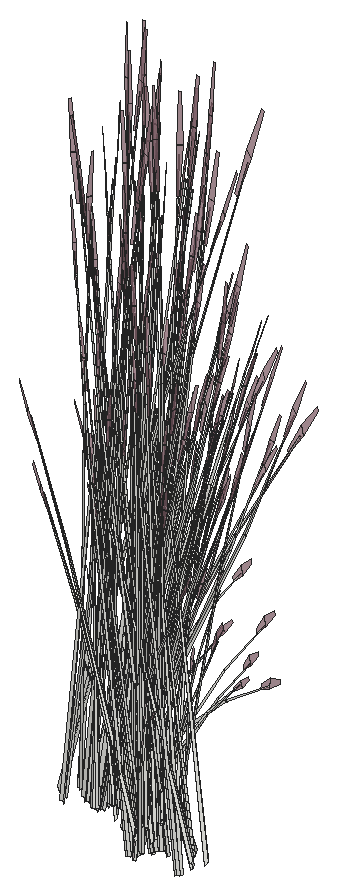
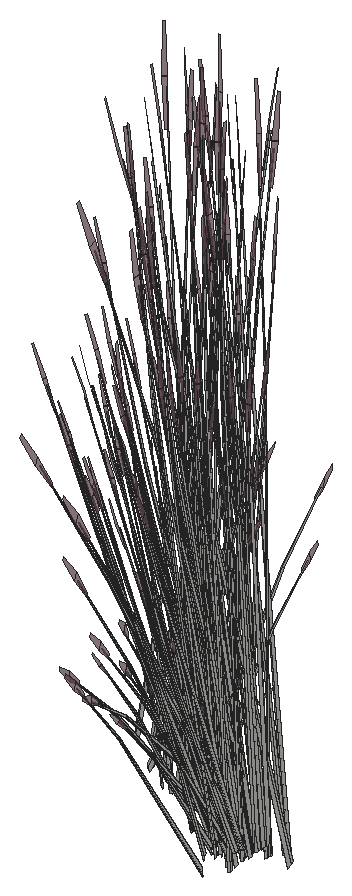
# SketchUp Ruby script. Lengths in inches.
U = 1.inch
M = Sketchup.active_model
def pt(a) = Geom::Point3d.new(a.map { |v| v * U })
def face(e, loops, mat)
  f = e.add_face(loops[0].map { |a| pt(a) })
  loops[1..].each { |l| e.add_face(l.map { |a| pt(a) }).erase! }
  f.material = f.back_material = mat if mat
  f
end
# faces: each face lists its corners as indices into pts; further lists are holes
def faces(e, pts, list, mat = nil) = list.each { |f| face(e, (f[0].is_a?(Array) ? f : [f]).map { |l| l.map { |i| pts[i] } }, mat) }
# xy, xz, yz: faces in a plane at the given z, y or x. An outline is a flat list of corners, or four numbers for a rectangle; further outlines are holes
def ring(l) = l.size == 4 ? [[l[0], l[1]], [l[2], l[1]], [l[2], l[3]], [l[0], l[3]]] : l.each_slice(2).to_a
def flat(e, list, mat, &to3) = list.each { |f| face(e, (f[0].is_a?(Array) ? f : [f]).map { |l| ring(l).map { |u, v| to3.(u, v) } }, mat) }
def xy(e, z, list, mat = nil) = flat(e, list, mat) { |x, y| [x, y, z] }
def xz(e, y, list, mat = nil) = flat(e, list, mat) { |x, z| [x, y, z] }
def yz(e, x, list, mat = nil) = flat(e, list, mat) { |y, z| [x, y, z] }
def lines(e, pts, list) = list.each { |a, b| e.add_line(pt(pts[a]), pt(pts[b])) }
# prism: a flat outline (further loops are holes) pulled along v
def prism(e, loops, v, mat = nil)
  f = face(e, loops, mat); d = Geom::Vector3d.new(v.map { |x| x * U })
  f.pushpull(f.normal.samedirection?(d) ? d.length : -d.length)
end
def box(e, o, s, mat = nil) = prism(e, [[o, [o[0] + s[0], o[1], o[2]], [o[0] + s[0], o[1] + s[1], o[2]], [o[0], o[1] + s[1], o[2]]]], [0, 0, s[2]], mat)
def at(x, y, z, deg = 0) = Geom::Transformation.translation(pt([x, y, z])) * Geom::Transformation.rotation(ORIGIN, Z_AXIS, deg.degrees)
def axes(o, x, y, z) = Geom::Transformation.new([*x, 0, *y, 0, *z, 0, *pt(o).to_a, 1])
def part(name) = M.definitions.add(name)
# library, detail: a bought-in or finely detailed component or shape, given as its bounding box
def library(name, o, s) = part(name).tap { |d| box(d.entities, o, s) }
def detail(e, o, s) = box(e.add_group.entities, o, s)
def put(e, d, t, mat = nil) = e.add_instance(d, t).tap { |i| i.material = mat if mat }
def group(e, t, mat = nil) = e.add_group.tap { |g| g.transformation = t; g.material = mat if mat }.entities
root = M.entities
M.materials.add("LightPink_Translucent").color = [144, 107, 117]
M.materials["LightPink_Translucent"].alpha = 0.75
c1 = part("blade")
p = [[2.15,0.21,22],[0,0.17,0],[0.09,0.45,0],[2.18,0.31,22],[2.29,0.31,22],[0.38,0.45,0],
  [2.48,0.24,33],[2.49,0.24,33],[2.48,0.22,33]]
faces(c1.entities,p,[[0,1,2,3],[4,5,2,3],[6,3,4,7],[8,0,3,6]])
c2 = part("seeds")
p = [[0.3,-0.1,1.38],[-0.01,-0.03,1.59],[-0.01,-0.03,0.03],[0.14,-0.07,-0.07],[0.29,-0.03,3],[0.15,0.01,3.11]]
faces(c2.entities,p,[[0,1,2,3],[1,0,4,5]],"LightPink_Translucent")
c3 = part("blade with seeds")
put(c3.entities,c1,at(0,0,0))
put(c3.entities,c2,axes([2.4,0.25,30.99],[1.5799,-0.05474,1.17369],[-0.12525,1.92788,0.29478],[-0.07173,-0.02425,1.56792]))
put(root,c3,axes([670.11,342.17,391.97],[-0.40676,0.57214,0],[-0.68052,-0.31907,-0.42834],[-0.15499,-0.07267,1.3588]))
put(root,c3,axes([663.61,345.16,394.18],[-0.60181,-0.31483,-0.10093],[0.34671,-0.45593,-0.56021],[0.17003,-0.15849,0.85122]))
put(root,c3,axes([668.6875,340.6,392.26],[0.70648,-0.03525,0.37133],[0.06389,0.58508,-0.17871],[-0.12647,0.0593,1.19224]))
put(root,c3,axes([668.06,340.89,391.83],[-0.70648,0.03525,-0.37133],[-0.06389,-0.58508,0.17871],[-0.12647,0.0593,1.19224]))
put(root,c3,axes([671.81,340.89,391.83],[-0.70648,0.03525,-0.37133],[-0.06389,-0.58508,0.17871],[-0.12647,0.0593,1.19224]))
put(root,c3,axes([660.2,343.6,391.67],[0.60889,-0.28548,-0.4121],[0.36394,0.51192,0],[0.13868,-0.06502,1.30728]))
put(root,c3,axes([663.82,344.58,392.15],[-0.23242,-0.01691,1.18691],[-0.23811,-0.45367,-0.25526],[0.28553,-0.12834,0.50747]))
put(root,c3,axes([665.09,345.02,393.91],[-0.08498,-0.00434,1.47228],[-0.35287,-0.46464,-0.13912],[0.14171,-0.15278,0.26054]))
put(root,c3,axes([660.93,344.77,391.71],[0.43821,-0.42916,-0.51753],[0.54436,0.38915,-0.13583],[0.1756,-0.10706,1.14236]))
put(root,c3,axes([664.09,343.75,392.3],[-0.2167,0.29065,0.95334],[-0.18626,-0.3905,0.70045],[0.17898,-0.09785,0.20998]))
put(root,c3,axes([668.84,342.25,391.82],[-0.40169,-0.57414,-0.04268],[0.68052,-0.31907,0.42834],[-0.16769,0.05466,1.35813]))
put(root,c3,axes([668.7,340.86,392.17],[0.48065,0.34305,0.12018],[-0.40092,0.38703,-0.34318],[-0.1116,0.05232,1.05198]))
put(root,c3,axes([668.65,340.95,393.93],[-0.16135,-0.52549,0.39842],[0.63294,-0.0912,0.32852],[-0.18654,0.12359,0.82444]))
put(root,c3,axes([668.53,340.85,393.93],[-0.44663,-0.24013,0.05337],[0.26003,-0.34195,0.42015],[-0.14319,0.11055,0.64067]))
put(root,c3,axes([668.73,340.21,393.22],[0.22574,-0.12077,1.42242],[0.19004,0.55807,0.11501],[-0.35439,0.12613,0.60807]))
put(root,c3,axes([672.91,340.21,393.22],[0.22574,-0.12077,1.42242],[0.19004,0.55807,0.11501],[-0.35439,0.12613,0.60807]))
put(root,c3,axes([663.78,344.84,393.76],[0.56631,-0.0816,-0.29394],[0.14954,0.46647,0.37948],[0.16229,-0.12529,0.72609]))
put(root,c3,axes([660.45,345.26,392.21],[-0.07581,-0.65151,-0.24149],[0.7896,-0.03939,-0.41502],[0.13904,-0.08678,1.32557]))
put(root,c3,axes([669.21,341.91,392.06],[0.60889,-0.28548,0.4121],[0.36394,0.51192,0],[-0.13868,0.06502,1.30728]))
put(root,c3,axes([663.3125,345.12,394.19],[-0.56631,0.0816,0.29394],[-0.14954,-0.46647,-0.37948],[0.16229,-0.12529,0.72609]))
put(root,c3,axes([668.35,341.46,391.9],[0.28286,0.65594,-0.0499],[-0.80821,0.22985,0],[0.00988,0.02291,1.42904]))
put(root,c3,axes([668.66,342.17,391.68],[-0.60696,-0.14127,-0.25712],[0.15283,-0.49751,0.25712],[-0.12236,0.05737,1.15348]))
put(root,c3,axes([668.03,341.16,392.15],[0.2261,0.04687,1.18691],[0.14573,0.47875,-0.25526],[-0.30712,0.08962,0.50747]))
put(root,c3,axes([672.21,341.16,392.15],[0.2261,0.04687,1.18691],[0.14573,0.47875,-0.25526],[-0.30712,0.08962,0.50747]))
put(root,c3,axes([665.29,340.77,394.19],[0.56631,-0.0816,0.29394],[0.14954,0.46647,-0.37948],[-0.16229,0.12529,0.72609]))
put(root,c3,axes([669.04,340.77,394.19],[0.56631,-0.0816,0.29394],[0.14954,0.46647,-0.37948],[-0.16229,0.12529,0.72609]))
put(root,c3,axes([666.86,340.5625,393.91],[0.08303,0.01531,1.47228],[0.25685,0.50448,-0.13912],[-0.16996,0.13241,0.26054]))
put(root,c3,axes([671.04,340.5625,393.91],[0.08303,0.01531,1.47228],[0.25685,0.50448,-0.13912],[-0.16996,0.13241,0.26054]))
put(root,c3,axes([660.35,343.82,391.68],[0.60696,0.14127,-0.25712],[-0.15283,0.49751,0.25712],[0.12236,-0.05737,1.15348]))
put(root,c3,axes([667.56,342.17,392.3],[0.27113,-0.25877,0.95334],[0.10699,0.40966,0.70045],[-0.19594,0.07335,0.20998]))
put(root,c3,axes([671.74,342.17,392.3],[0.27113,-0.25877,0.95334],[0.10699,0.40966,0.70045],[-0.19594,0.07335,0.20998]))
put(root,c3,axes([668.56,340.73,392.21],[0.07581,0.65151,-0.24149],[-0.7896,0.03939,-0.41502],[-0.13904,0.08678,1.32557]))
put(root,c3,axes([668.84,340.48,391.83],[-0.31565,0.51449,-0.37133],[-0.65588,-0.24761,0.17871],[0,0.1186,1.19224]))
put(root,c3,axes([668.58,341.05,393.76],[-0.56631,0.0816,-0.29394],[-0.14954,-0.46647,0.37948],[-0.16229,0.12529,0.72609]))
put(root,c3,axes([672.76,341.05,393.76],[-0.56631,0.0816,-0.29394],[-0.14954,-0.46647,0.37948],[-0.16229,0.12529,0.72609]))
put(root,c3,axes([663.83,345.04,393.93],[0.44663,0.24013,0.05337],[-0.26003,0.34195,0.42015],[0.14319,-0.11055,0.64067]))
put(root,c3,axes([663.7,344.94,393.93],[0.16135,0.52549,0.39842],[-0.63294,0.0912,0.32852],[0.18654,-0.12359,0.82444]))
put(root,c3,axes([664.01,342.1,394.6875],[0.5741,0.15241,-0.05385],[-0.1766,0.46909,-0.24415],[-0.0939,0.07122,0.8053]))
put(root,c3,axes([667.76,342.1,394.6875],[0.5741,0.15241,-0.05385],[-0.1766,0.46909,-0.24415],[-0.0939,0.07122,0.8053]))
put(root,c3,axes([668.08,341.23,391.71],[-0.43821,0.42916,-0.51753],[-0.54436,-0.38915,-0.13583],[-0.1756,0.10706,1.14236]))
put(root,c3,axes([671.83,341.23,391.71],[-0.43821,0.42916,-0.51753],[-0.54436,-0.38915,-0.13583],[-0.1756,0.10706,1.14236]))
put(root,c3,axes([668.86,341.95,391.93],[0.81449,0.18558,0.25528],[-0.20377,0.66335,-0.30288],[-0.13481,0.08302,1.36855]))
put(root,c3,axes([668.8,342.4,391.67],[-0.60889,0.28548,-0.4121],[-0.36394,-0.51192,0],[-0.13868,0.06502,1.30728]))
put(root,c3,axes([665,340.73,394.18],[0.60181,0.31483,-0.10093],[-0.34671,0.45593,-0.56021],[-0.17003,0.15849,0.85122]))
put(root,c3,axes([668.75,340.73,394.18],[0.60181,0.31483,-0.10093],[-0.34671,0.45593,-0.56021],[-0.17003,0.15849,0.85122]))
put(root,c3,axes([669.56,340.59,393.22],[0.1625,-0.17544,1.42242],[0.41029,0.47354,0.11501],[-0.28141,0.21565,0.60807]))
put(root,c3,axes([673.74,340.59,393.22],[0.1625,-0.17544,1.42242],[0.41029,0.47354,0.11501],[-0.28141,0.21565,0.60807]))
put(root,c3,axes([663.63,346.39,394.18],[-0.32734,-0.51701,-0.10093],[0.58097,-0.25407,-0.56021],[0.24483,-0.06821,0.85122]))
put(root,c3,axes([663.6,345.94,393.89],[0.17625,-0.51936,-0.42412],[0.60429,0.17802,-0.32852],[0.2433,-0.04762,0.81151]))
put(root,c3,axes([662.65,343.83,391.97],[0.40676,-0.57214,0],[0.68052,0.31907,-0.42834],[0.15499,0.07267,1.3588]))
put(root,c3,axes([669.05,341.1,393.89],[0.16713,0.52135,-0.42412],[-0.63294,0.0912,-0.32852],[-0.18138,0.14003,0.81151]))
put(root,c3,axes([666.06,341.7,394.19],[0.4402,-0.30062,0.29394],[0.41671,0.34326,-0.37948],[-0.0634,0.1744,0.72609]))
put(root,c3,axes([669.35,342.31,391.97],[0.40676,0.57214,0],[-0.68052,0.31907,-0.42834],[-0.15499,0.07267,1.3588]))
put(root,c3,axes([664.25,346.09,391.65],[-0.41902,0.06852,1.17514],[-0.0667,-0.54541,0.06726],[0.29348,-0.08255,0.6687]))
put(root,c3,axes([665.01,345.61,391.875],[-0.40335,-0.3651,-0.05385],[0.44175,-0.33453,-0.24415],[0.12517,-0.02355,0.8053]))
put(root,c3,axes([669.01,340.04,392.36],[-0.01777,-0.53759,1.17256],[0.80434,0.13935,0.49647],[-0.19024,0.29416,1.1068]))
put(root,c3,axes([665.66,341.97,393.93],[-0.53464,-0.0266,0.05337],[0.01466,-0.40172,0.42015],[-0.05594,0.15388,0.64067]))
put(root,c3,axes([669.41,341.97,393.93],[-0.53464,-0.0266,0.05337],[0.01466,-0.40172,0.42015],[-0.05594,0.15388,0.64067]))
put(root,c3,axes([668.27,342.43,391.24],[0.08727,0.05704,1.46364],[0.14797,0.52853,-0.2236],[-0.19341,0.11271,0.24931]))
put(root,c3,axes([665.83,342.01,393.93],[-0.46327,-0.38957,0.39842],[0.49199,-0.33598,0.32852],[-0.08546,0.18277,0.82444]))
put(root,c3,axes([669.58,342.01,393.93],[-0.46327,-0.38957,0.39842],[0.49199,-0.33598,0.32852],[-0.08546,0.18277,0.82444]))
put(root,c3,axes([662.3,344.13,392.06],[-0.60889,-0.28548,0.4121],[0.36394,-0.51192,0],[0.13868,0.06502,1.30728]))
put(root,c3,axes([667.29,342.2,394.19],[0.19614,-0.43908,0.29394],[0.57222,0.12807,-0.37948],[0.05247,0.17678,0.72609]))
put(root,c3,axes([660.92,345.24,391.96],[-0.53943,0.51816,0.37976],[-0.64086,-0.4574,0.14902],[0.13005,-0.05171,1.31851]))
put(root,c3,axes([663.4,346.23,394.19],[-0.54068,-0.15928,0.29394],[0.1577,-0.46469,-0.37948],[0.21769,-0.04261,0.72609]))
put(root,c3,axes([659.7,344.84,391.32],[-0.64037,0.22859,1.07011],[-0.20382,-0.65589,0.4158],[0.39323,0.01091,1.21713]))
put(root,c3,axes([661.42,345.02,392.17],[0.12551,-0.50956,0.12018],[0.6132,0.08845,-0.34318],[0.1116,0.05232,1.05198]))
put(root,c3,axes([669.4375,341.02,393.22],[0.12114,-0.19625,1.42242],[0.50818,0.40613,0.11501],[-0.22925,0.25313,0.60807]))
put(root,c3,axes([661.16,345.15,392.26],[-0.39083,-0.47924,0.37133],[0.59199,-0.33747,-0.17871],[0.12647,0.0593,1.19224]))
put(root,c3,axes([667.11,342.59,393.93],[-0.47939,0.19405,0.05337],[-0.23464,-0.35385,0.42015],[0.0463,0.15598,0.64067]))
put(root,c3,axes([665.83,342.13,393.76],[-0.4402,0.30062,-0.29394],[-0.41671,-0.34326,0.37948],[-0.0634,0.1744,0.72609]))
put(root,c3,axes([669.58,342.13,393.76],[-0.4402,0.30062,-0.29394],[-0.41671,-0.34326,0.37948],[-0.0634,0.1744,0.72609]))
put(root,c3,axes([668.06,342.04,393.91],[-0.01617,0.11299,1.45204],[0.45894,0.39307,-0.22964],[-0.12015,0.18588,0.11645]))
put(root,c3,axes([665.78,341.78,394.48],[0.71502,0.02829,-0.11203],[-0.01954,0.53563,-0.62183],[-0.04967,0.20629,0.94486]))
put(root,c3,axes([661.36,345.18,392.21],[0.65687,-0.37907,-0.24149],[0.43681,0.53562,-0.41502],[0.16207,0.0544,1.32557]))
put(root,c3,axes([667.28,342.56,394.2],[-0.64106,-0.14927,0.44225],[0.21921,-0.49074,0.36465],[0.03852,0.19299,0.91512]))
put(root,c3,axes([663.97,346.18,393.76],[0.54068,0.15928,-0.29394],[-0.1577,0.46469,0.37948],[0.21769,-0.04261,0.72609]))
put(root,c3,axes([666.11,343.3,392.3],[-0.01684,-0.3395,0.95334],[0.42072,0.24214,0.70045],[-0.08274,0.16182,0.20998]))
put(root,c3,axes([669.86,343.3,392.3],[-0.01684,-0.3395,0.95334],[0.42072,0.24214,0.70045],[-0.08274,0.16182,0.20998]))
put(root,c3,axes([663.02,344.17,391.67],[0.60889,0.28548,-0.4121],[-0.36394,0.51192,0],[0.13868,0.06502,1.30728]))
put(root,c3,axes([661.86,345.8,391.83],[0.72788,0,0],[0,0.59111,0],[0,0,1.48078]))
put(root,c3,axes([667.22,342.48,391.24],[0.10529,-0.03107,1.46364],[0.63335,0.17101,-0.2236],[0.01852,0.19274,0.24931]))
put(root,c3,axes([666.27,341.99,394.15],[0.46573,0.38364,-0.47077],[-0.49199,0.33598,-0.36465],[-0.07086,0.19492,0.90078]))
put(root,c3,axes([662.85,344.39,391.68],[0.15283,0.49751,-0.25712],[-0.60696,0.14127,0.25712],[0.12236,0.05737,1.15348]))
put(root,c3,axes([665.76,342.5625,392.34],[0.59102,-0.10111,0.05401],[0.13587,0.40735,-0.71633],[-0.03747,0.2062,0.64209]))
put(root,c3,axes([663.89,346.375,393.93],[0.23895,0.38931,0.05337],[-0.43573,0.19055,0.42015],[0.19208,-0.0376,0.64067]))
put(root,c3,axes([661.625,345.5,391.98],[-0.82229,-0.1203,0.40835],[0.16734,-0.67942,0.16024],[0.12017,0.06561,1.41775]))
put(root,c3,axes([663.85,346.24,393.93],[-0.18381,0.5206,0.39842],[-0.60429,-0.17802,0.32852],[0.23764,-0.03129,0.82444]))
put(root,c3,axes([667.36,342.66,393.76],[-0.19614,0.43908,-0.29394],[-0.57222,-0.12807,0.37948],[0.05247,0.17678,0.72609]))
put(root,c3,axes([661.77,347.11,391.8125],[0.68303,-0.19373,-0.15934],[0.24001,0.55805,0.00007],[0.07539,-0.02141,1.44335]))
put(root,c3,axes([666.12,341.81,394.43],[-0.01693,0.52814,-0.65454],[-0.71285,-0.03547,0.07899],[-0.07523,0.22375,0.92591]))
put(root,c3,axes([669.87,341.81,394.43],[-0.01693,0.52814,-0.65454],[-0.71285,-0.03547,0.07899],[-0.07523,0.22375,0.92591]))
put(root,c3,axes([664.26,343.2,393.91],[0.07381,-0.03447,1.47228],[0.61004,0.22929,-0.13912],[-0.01434,0.19091,0.26054]))
put(root,c3,axes([668.01,343.2,393.91],[0.07381,-0.03447,1.47228],[0.61004,0.22929,-0.13912],[-0.01434,0.19091,0.26054]))
put(root,c3,axes([661.85,346.06,391.84],[0.45414,0.3688,0],[-0.45414,0.3688,0],[0,0,1.40491]))
put(root,c3,axes([662.13,345.27,391.71],[0.67676,0.09361,-0.51753],[-0.14281,0.57742,-0.13583],[0.20196,0.06997,1.14236]))
put(root,c3,axes([666.8,341.44,393.22],[-0.01592,-0.21915,1.42242],[0.69015,0.14538,0.11501],[-0.04269,0.3123,0.60807]))
put(root,c3,axes([665.12,346.27,392.3],[-0.40197,0.09426,0.95334],[0.18921,-0.38956,0.70045],[0.21325,0.02666,0.20998]))
put(root,c3,axes([661.84,345.625,392.26],[0.31565,-0.51449,0.37133],[0.65588,0.24761,-0.17871],[0,0.1186,1.19224]))
put(root,c3,axes([665.62,342.99,392.15],[0.2053,-0.09007,1.18691],[0.50689,0.27159,-0.25526],[-0.15087,0.235,0.50747]))
put(root,c3,axes([669.37,342.99,392.15],[0.2053,-0.09007,1.18691],[0.50689,0.27159,-0.25526],[-0.15087,0.235,0.50747]))
put(root,c3,axes([666.95,343.4375,393.91],[0.08247,0.09194,1.45204],[0.66552,0.03612,-0.22964],[0.06692,0.20277,0.11645]))
put(root,c3,axes([661.78,345.45,391.83],[0.39083,0.47924,-0.37133],[-0.59199,0.33747,0.17871],[0.12647,0.0593,1.19224]))
put(root,c3,axes([664.42,347.48,393.26],[-0.12452,-0.47997,-0.02898],[0.58854,-0.11034,-0.1314],[0.1229,0.03043,0.43341]))
put(root,c3,axes([662.9,347.46,394.18],[0.03484,-0.58066,-0.10093],[0.65957,0.01587,-0.56021],[0.25402,0.04034,0.85122]))
put(root,c3,axes([663.5,345.91,392.06],[0,-0.57097,0.4121],[0.72788,0,0],[0,0.13004,1.30728]))
put(root,c3,axes([662.11,345.74,392.17],[0.60616,-0.16651,0.12018],[0.21227,0.47548,-0.34318],[0,0.10465,1.05198]))
put(root,c3,axes([662.79,347.23,394.19],[-0.37017,-0.35748,0.29394],[0.42268,-0.3384,-0.37948],[0.21476,0.05149,0.72609]))
put(root,c3,axes([665.88,342.55,392.79],[0.01429,-0.29475,1.28107],[0.64291,0.15569,0.17703],[-0.0557,0.31414,0.60492]))
put(root,c3,axes([669.63,342.55,392.79],[0.01429,-0.29475,1.28107],[0.64291,0.15569,0.17703],[-0.0557,0.31414,0.60492]))
put(root,c3,axes([661.57,347.41,391.83],[0.65588,0.25634,0],[-0.31565,0.53263,0],[0,0,1.45212]))
put(root,c3,axes([663.47,347.11,393.91],[0.13956,-0.00966,1.45204],[0.38281,-0.44358,-0.22964],[0.24825,0.05855,0.11645]))
put(root,c3,axes([662.93,347.18,394.13],[0.65035,0.01375,-0.58968],[-0.04368,0.5789,0.07116],[0.27552,0.06109,0.83415]))
put(root,c3,axes([663.99,346.01,391.97],[0.81352,0,0],[0,0.63814,-0.42834],[0,0.14534,1.3588]))
put(root,c3,axes([661.91,345.78,392.21],[0.73268,0.27244,-0.24149],[-0.35279,0.57501,-0.41502],[0.02303,0.14118,1.32557]))
put(root,c3,axes([663.32,347.42,393.76],[0.37017,0.35748,-0.29394],[-0.42268,0.3384,0.37948],[0.21476,0.05149,0.72609]))
put(root,c3,axes([663.5,346.43,391.68],[-0.45414,0.35624,-0.25712],[-0.45414,-0.35624,0.25712],[0,0.11474,1.15348]))
put(root,c3,axes([663.13,347.56,393.93],[-0.03276,0.43418,0.05337],[-0.49468,-0.0119,0.42015],[0.18949,0.04543,0.64067]))
put(root,c3,axes([663.18,347.42,393.93],[-0.47971,0.37622,0.39842],[-0.41372,-0.39954,0.32852],[0.22506,0.0694,0.82444]))
put(root,c3,axes([661.65,347.85,394.19],[-0.10048,-0.4599,0.29394],[0.5744,-0.12144,-0.37948],[0.15428,0.13179,0.72609]))
put(root,c3,axes([663.81,346.44,391.67],[0,0.57097,-0.4121],[-0.72788,0,0],[0,0.13004,1.30728]))
put(root,c3,axes([661.99,346.5,393.22],[-0.24166,-0.09837,1.42242],[0.50011,-0.41269,0.11501],[0.3117,0.18617,0.60807]))
put(root,c3,axes([662.04,345.21,393.71],[-0.56218,-0.29666,1.14775],[0.59361,-0.46189,0.49522],[0.18138,0.27836,1.10941]))
put(root,c3,axes([662.88,347.625,392.3],[-0.36631,-0.16417,0.95334],[0.47299,-0.16681,0.70045],[0.12758,0.1413,0.20998]))
put(root,c3,axes([661.6,348.09,394.18],[0.38768,-0.48872,-0.10093],[0.56143,0.28156,-0.56021],[0.19516,0.13808,0.85122]))
put(root,c3,axes([661.09,348.5,393.91],[0.00193,-0.06913,1.47228],[0.55753,-0.30498,-0.13912],[0.19366,0.10886,0.26054]))
put(root,c3,axes([662.99,348.23,391.24],[0.0474,-0.08243,1.46364],[0.59674,-0.24277,-0.2236],[0.18092,0.12565,0.24931]))
put(root,c3,axes([662.2,346.36,391.74],[0.23855,0.52277,-0.57446],[-0.68718,0.18827,-0.15077],[0.02637,0.17702,1.26801]))
put(root,c3,axes([662.06,347.85,393.89],[0.64198,-0.13573,-0.42412],[0.1123,0.514,-0.32852],[0.17243,0.1473,0.81151]))
put(root,c3,axes([662.94,348.37,392.21],[-0.4172,-0.01791,0.872],[0.27552,-0.38032,0.48145],[0.16481,0.13512,0.68401]))
put(root,c3,axes([661.74,348.27,393.93],[-0.29569,0.36271,0.05337],[-0.42107,-0.21117,0.42015],[0.13613,0.11629,0.64067]))
put(root,c3,axes([661.05,349.49,394.6875],[0.44958,-0.32756,-0.05385],[0.41194,0.35875,-0.24415],[0.029,0.10165,0.8053]))
put(root,c3,axes([661.87,348.17,393.93],[-0.64708,0.13103,0.39842],[-0.1123,-0.514,0.32852],[0.15218,0.15149,0.82444]))
put(root,c3,axes([661.58,347.45,392.15],[0.01148,-0.18927,1.18691],[0.54864,-0.21141,-0.25526],[0.16937,0.22654,0.50747]))
put(root,c3,axes([660.08,348.11,394.18],[0.63664,-0.26583,-0.10093],[0.31286,0.47181,-0.56021],[0.084,0.19882,0.85122]))
put(root,c3,axes([660.63,348.09,393.89],[0.63954,0.14313,-0.42412],[-0.21921,0.49074,-0.32852],[0.05864,0.19758,0.81151]))
put(root,c3,axes([660.99,347.08,393.22],[-0.14872,-0.18332,1.42242],[0.6872,-0.15433,0.11501],[0.15531,0.28779,0.60807]))
